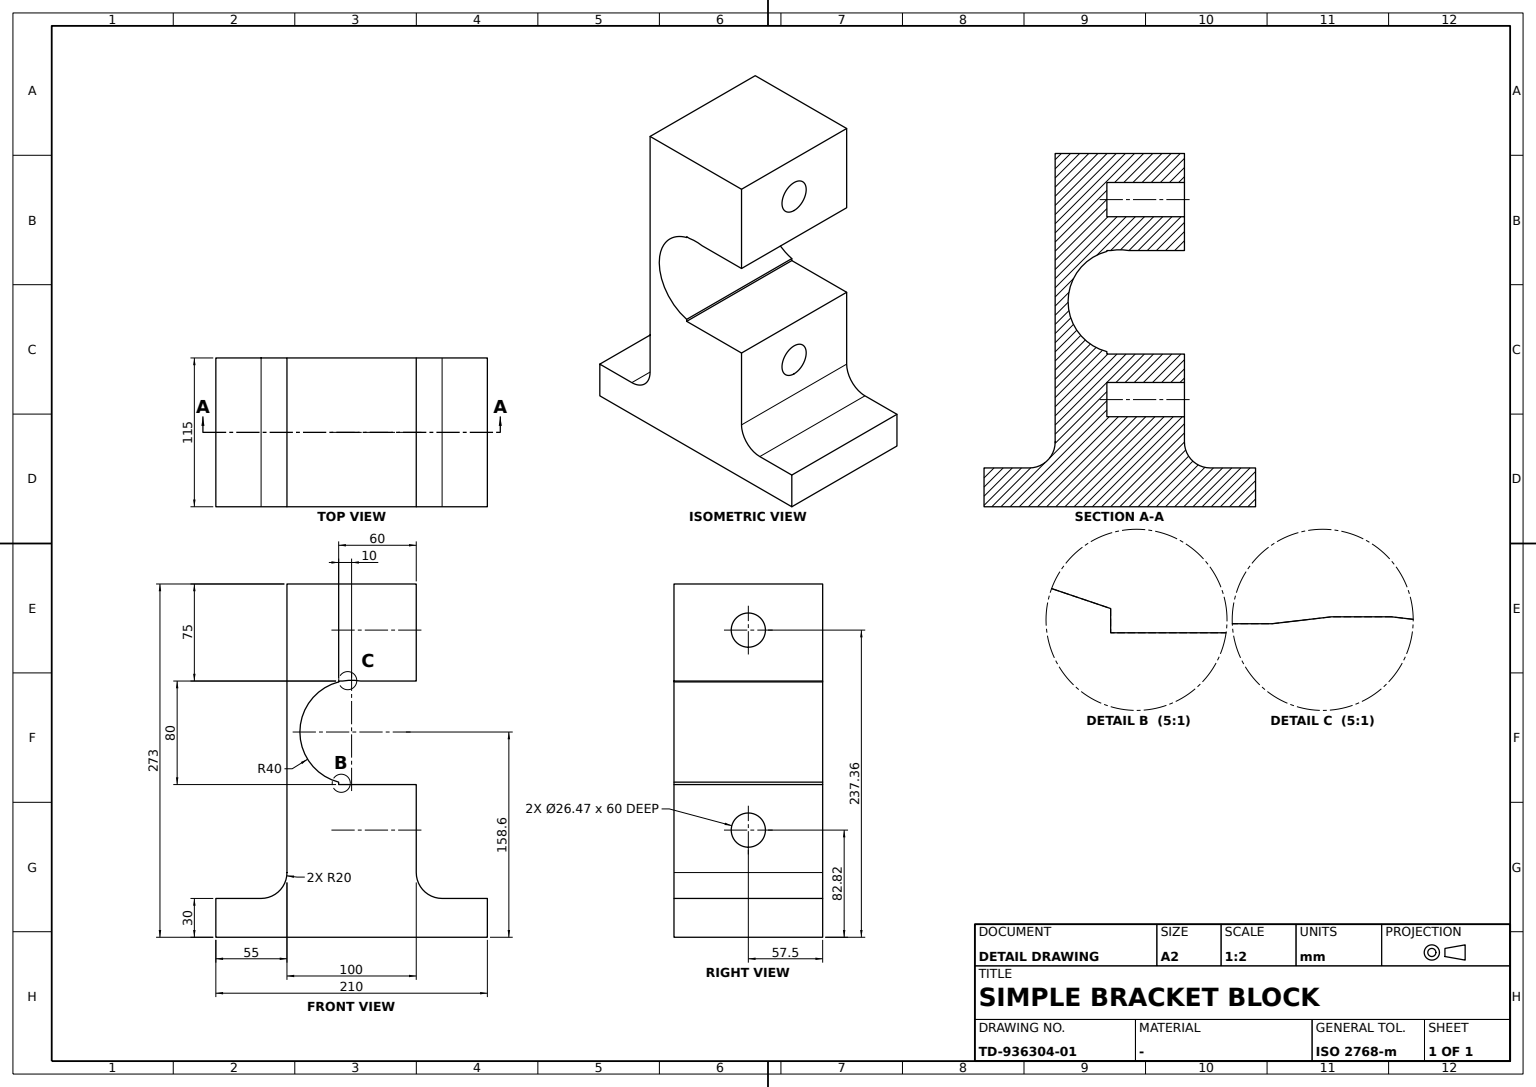
ISO-10303-21;
HEADER;
FILE_DESCRIPTION((''),'2;1');
FILE_NAME('','',(''),(''),'','','');
FILE_SCHEMA(('AUTOMOTIVE_DESIGN'));
ENDSEC;
DATA;
#1=APPLICATION_CONTEXT('');
#2=PRODUCT_CONTEXT('',#1,'mechanical');
#3=PRODUCT('','','',(#2));
#4=PRODUCT_DEFINITION_FORMATION('','',#3);
#5=PRODUCT_DEFINITION_CONTEXT('',#1,'design');
#6=PRODUCT_DEFINITION('','',#4,#5);
#7=PRODUCT_DEFINITION_SHAPE('','',#6);
#8=(LENGTH_UNIT()NAMED_UNIT(*)SI_UNIT(.MILLI.,.METRE.));
#9=(NAMED_UNIT(*)PLANE_ANGLE_UNIT()SI_UNIT($,.RADIAN.));
#10=(NAMED_UNIT(*)SI_UNIT($,.STERADIAN.)SOLID_ANGLE_UNIT());
#11=UNCERTAINTY_MEASURE_WITH_UNIT(LENGTH_MEASURE(0.005),#8,'distance_accuracy_value','');
#12=(GEOMETRIC_REPRESENTATION_CONTEXT(3)GLOBAL_UNCERTAINTY_ASSIGNED_CONTEXT((#11))GLOBAL_UNIT_ASSIGNED_CONTEXT((#8,#9,#10))REPRESENTATION_CONTEXT('',''));
#13=CARTESIAN_POINT('',(50.,57.5,118.));
#14=VERTEX_POINT('',#13);
#15=CARTESIAN_POINT('',(-10.,57.5,118.));
#16=VERTEX_POINT('',#15);
#17=DIRECTION('',(-1.,0.,0.));
#18=VECTOR('',#17,1000.);
#19=LINE('',#13,#18);
#20=EDGE_CURVE('',#14,#16,#19,.T.);
#21=ORIENTED_EDGE('',*,*,#20,.T.);
#22=CARTESIAN_POINT('',(-10.,-57.5,118.));
#23=VERTEX_POINT('',#22);
#24=DIRECTION('',(0.,-1.,0.));
#25=VECTOR('',#24,1000.);
#26=LINE('',#15,#25);
#27=EDGE_CURVE('',#16,#23,#26,.T.);
#28=ORIENTED_EDGE('',*,*,#27,.T.);
#29=CARTESIAN_POINT('',(50.,-57.5,118.));
#30=VERTEX_POINT('',#29);
#31=CARTESIAN_POINT('',(105.,-57.5,118.));
#32=LINE('',#31,#18);
#33=EDGE_CURVE('',#30,#23,#32,.T.);
#34=ORIENTED_EDGE('',*,*,#33,.F.);
#35=LINE('',#13,#25);
#36=EDGE_CURVE('',#14,#30,#35,.T.);
#37=ORIENTED_EDGE('',*,*,#36,.F.);
#38=EDGE_LOOP('',(#21,#28,#34,#37));
#39=FACE_BOUND('',#38,.T.);
#40=DIRECTION('',(0.,0.,-1.));
#41=AXIS2_PLACEMENT_3D('',#13,#40,#24);
#42=PLANE('',#41);
#43=ADVANCED_FACE('',(#39),#42,.F.);
#44=CARTESIAN_POINT('',(-105.,-57.5,0.));
#45=VERTEX_POINT('',#44);
#46=CARTESIAN_POINT('',(-105.,57.5,0.));
#47=VERTEX_POINT('',#46);
#48=CARTESIAN_POINT('',(-105.,0.,0.));
#49=DIRECTION('',(0.,1.,0.));
#50=VECTOR('',#49,1000.);
#51=LINE('',#48,#50);
#52=EDGE_CURVE('',#45,#47,#51,.T.);
#53=ORIENTED_EDGE('',*,*,#52,.F.);
#54=CARTESIAN_POINT('',(-105.,-57.5,30.));
#55=VERTEX_POINT('',#54);
#56=DIRECTION('',(0.,0.,1.));
#57=VECTOR('',#56,1000.);
#58=LINE('',#44,#57);
#59=EDGE_CURVE('',#45,#55,#58,.T.);
#60=ORIENTED_EDGE('',*,*,#59,.T.);
#61=CARTESIAN_POINT('',(-105.,57.5,30.));
#62=VERTEX_POINT('',#61);
#63=CARTESIAN_POINT('',(-105.,0.,30.));
#64=LINE('',#63,#50);
#65=EDGE_CURVE('',#55,#62,#64,.T.);
#66=ORIENTED_EDGE('',*,*,#65,.T.);
#67=LINE('',#46,#57);
#68=EDGE_CURVE('',#47,#62,#67,.T.);
#69=ORIENTED_EDGE('',*,*,#68,.F.);
#70=EDGE_LOOP('',(#53,#60,#66,#69));
#71=FACE_BOUND('',#70,.T.);
#72=DIRECTION('',(1.,0.,0.));
#73=AXIS2_PLACEMENT_3D('',#44,#72,#49);
#74=PLANE('',#73);
#75=ADVANCED_FACE('',(#71),#74,.F.);
#76=CARTESIAN_POINT('',(-50.,-57.5,50.));
#77=VERTEX_POINT('',#76);
#78=CARTESIAN_POINT('',(-50.,57.5,50.));
#79=VERTEX_POINT('',#78);
#80=CARTESIAN_POINT('',(-50.,0.,50.));
#81=LINE('',#80,#50);
#82=EDGE_CURVE('',#77,#79,#81,.T.);
#83=ORIENTED_EDGE('',*,*,#82,.F.);
#84=CARTESIAN_POINT('',(-50.,-57.5,273.));
#85=VERTEX_POINT('',#84);
#86=CARTESIAN_POINT('',(-50.,-57.5,30.));
#87=LINE('',#86,#57);
#88=EDGE_CURVE('',#77,#85,#87,.T.);
#89=ORIENTED_EDGE('',*,*,#88,.T.);
#90=CARTESIAN_POINT('',(-50.,57.5,273.));
#91=VERTEX_POINT('',#90);
#92=CARTESIAN_POINT('',(-50.,0.,273.));
#93=LINE('',#92,#50);
#94=EDGE_CURVE('',#85,#91,#93,.T.);
#95=ORIENTED_EDGE('',*,*,#94,.T.);
#96=CARTESIAN_POINT('',(-50.,57.5,0.));
#97=LINE('',#96,#57);
#98=EDGE_CURVE('',#79,#91,#97,.T.);
#99=ORIENTED_EDGE('',*,*,#98,.F.);
#100=EDGE_LOOP('',(#83,#89,#95,#99));
#101=FACE_BOUND('',#100,.T.);
#102=AXIS2_PLACEMENT_3D('',#86,#72,#49);
#103=PLANE('',#102);
#104=ADVANCED_FACE('',(#101),#103,.F.);
#105=CARTESIAN_POINT('',(50.,57.5,50.));
#106=VERTEX_POINT('',#105);
#107=CARTESIAN_POINT('',(70.,57.5,30.));
#108=VERTEX_POINT('',#107);
#109=CARTESIAN_POINT('',(70.,57.5,50.));
#110=AXIS2_PLACEMENT_3D('',#109,#24,#40);
#111=CIRCLE('',#110,20.);
#112=EDGE_CURVE('',#106,#108,#111,.T.);
#113=ORIENTED_EDGE('',*,*,#112,.F.);
#114=CARTESIAN_POINT('',(50.,-57.5,50.));
#115=VERTEX_POINT('',#114);
#116=CARTESIAN_POINT('',(50.,0.,50.));
#117=LINE('',#116,#25);
#118=EDGE_CURVE('',#106,#115,#117,.T.);
#119=ORIENTED_EDGE('',*,*,#118,.T.);
#120=CARTESIAN_POINT('',(70.,-57.5,30.));
#121=VERTEX_POINT('',#120);
#122=CARTESIAN_POINT('',(70.,-57.5,50.));
#123=AXIS2_PLACEMENT_3D('',#122,#49,#56);
#124=CIRCLE('',#123,20.);
#125=EDGE_CURVE('',#121,#115,#124,.T.);
#126=ORIENTED_EDGE('',*,*,#125,.F.);
#127=CARTESIAN_POINT('',(70.,0.,30.));
#128=LINE('',#127,#25);
#129=EDGE_CURVE('',#108,#121,#128,.T.);
#130=ORIENTED_EDGE('',*,*,#129,.F.);
#131=EDGE_LOOP('',(#113,#119,#126,#130));
#132=FACE_BOUND('',#131,.T.);
#133=CARTESIAN_POINT('',(70.,0.,50.));
#134=AXIS2_PLACEMENT_3D('',#133,#24,#40);
#135=CYLINDRICAL_SURFACE('',#134,20.);
#136=ADVANCED_FACE('',(#132),#135,.F.);
#137=CARTESIAN_POINT('',(6.915696,-57.5,198.));
#138=VERTEX_POINT('',#137);
#139=CARTESIAN_POINT('',(6.915696,57.5,198.));
#140=VERTEX_POINT('',#139);
#141=LINE('',#139,#50);
#142=EDGE_CURVE('',#138,#140,#141,.T.);
#143=ORIENTED_EDGE('',*,*,#142,.F.);
#144=CARTESIAN_POINT('',(-6.915696,-57.5,198.));
#145=VERTEX_POINT('',#144);
#146=CARTESIAN_POINT('',(0.,-57.5,158.602371));
#147=AXIS2_PLACEMENT_3D('',#146,#49,#56);
#148=CIRCLE('',#147,40.);
#149=EDGE_CURVE('',#145,#138,#148,.T.);
#150=ORIENTED_EDGE('',*,*,#149,.F.);
#151=CARTESIAN_POINT('',(-6.915696,57.5,198.));
#152=VERTEX_POINT('',#151);
#153=LINE('',#151,#50);
#154=EDGE_CURVE('',#152,#145,#153,.F.);
#155=ORIENTED_EDGE('',*,*,#154,.F.);
#156=CARTESIAN_POINT('',(0.,57.5,158.602371));
#157=AXIS2_PLACEMENT_3D('',#156,#24,#40);
#158=CIRCLE('',#157,40.);
#159=EDGE_CURVE('',#152,#140,#158,.F.);
#160=ORIENTED_EDGE('',*,*,#159,.T.);
#161=EDGE_LOOP('',(#143,#150,#155,#160));
#162=FACE_BOUND('',#161,.T.);
#163=CARTESIAN_POINT('',(0.,-0.66,158.602371));
#164=AXIS2_PLACEMENT_3D('',#163,#49,#17);
#165=CYLINDRICAL_SURFACE('',#164,40.);
#166=ADVANCED_FACE('',(#162),#165,.F.);
#167=ORIENTED_EDGE('',*,*,#129,.T.);
#168=CARTESIAN_POINT('',(105.,-57.5,30.));
#169=VERTEX_POINT('',#168);
#170=CARTESIAN_POINT('',(0.,-57.5,30.));
#171=LINE('',#170,#18);
#172=EDGE_CURVE('',#169,#121,#171,.T.);
#173=ORIENTED_EDGE('',*,*,#172,.F.);
#174=CARTESIAN_POINT('',(105.,57.5,30.));
#175=VERTEX_POINT('',#174);
#176=CARTESIAN_POINT('',(105.,0.,30.));
#177=LINE('',#176,#25);
#178=EDGE_CURVE('',#175,#169,#177,.T.);
#179=ORIENTED_EDGE('',*,*,#178,.F.);
#180=CARTESIAN_POINT('',(0.,57.5,30.));
#181=VECTOR('',#72,1000.);
#182=LINE('',#180,#181);
#183=EDGE_CURVE('',#108,#175,#182,.T.);
#184=ORIENTED_EDGE('',*,*,#183,.F.);
#185=EDGE_LOOP('',(#167,#173,#179,#184));
#186=FACE_BOUND('',#185,.T.);
#187=CARTESIAN_POINT('',(0.,0.,30.));
#188=AXIS2_PLACEMENT_3D('',#187,#56,#72);
#189=PLANE('',#188);
#190=ADVANCED_FACE('',(#186),#189,.T.);
#191=CARTESIAN_POINT('',(-10.,0.,224.12904));
#192=VERTEX_POINT('',#191);
#193=CARTESIAN_POINT('',(-10.,0.,237.361694));
#194=AXIS2_PLACEMENT_3D('',#193,#72,#40);
#195=CIRCLE('',#194,13.232654);
#196=EDGE_CURVE('',#192,#192,#195,.T.);
#197=ORIENTED_EDGE('',*,*,#196,.T.);
#198=EDGE_LOOP('',(#197));
#199=FACE_BOUND('',#198,.T.);
#200=CARTESIAN_POINT('',(-10.,0.,0.));
#201=AXIS2_PLACEMENT_3D('',#200,#72,#49);
#202=PLANE('',#201);
#203=ADVANCED_FACE('',(#199),#202,.T.);
#204=CARTESIAN_POINT('',(-70.,-57.5,30.));
#205=VERTEX_POINT('',#204);
#206=CARTESIAN_POINT('',(-70.,57.5,30.));
#207=VERTEX_POINT('',#206);
#208=CARTESIAN_POINT('',(-70.,0.,30.));
#209=LINE('',#208,#50);
#210=EDGE_CURVE('',#205,#207,#209,.T.);
#211=ORIENTED_EDGE('',*,*,#210,.T.);
#212=EDGE_CURVE('',#62,#207,#182,.T.);
#213=ORIENTED_EDGE('',*,*,#212,.F.);
#214=ORIENTED_EDGE('',*,*,#65,.F.);
#215=EDGE_CURVE('',#205,#55,#171,.T.);
#216=ORIENTED_EDGE('',*,*,#215,.F.);
#217=EDGE_LOOP('',(#211,#213,#214,#216));
#218=FACE_BOUND('',#217,.T.);
#219=ADVANCED_FACE('',(#218),#189,.T.);
#220=CARTESIAN_POINT('',(50.,0.,250.594349));
#221=VERTEX_POINT('',#220);
#222=CARTESIAN_POINT('',(50.,0.,237.361694));
#223=AXIS2_PLACEMENT_3D('',#222,#17,#56);
#224=CIRCLE('',#223,13.232654);
#225=EDGE_CURVE('',#221,#221,#224,.F.);
#226=ORIENTED_EDGE('',*,*,#225,.T.);
#227=EDGE_LOOP('',(#226));
#228=FACE_BOUND('',#227,.T.);
#229=ORIENTED_EDGE('',*,*,#196,.F.);
#230=EDGE_LOOP('',(#229));
#231=FACE_BOUND('',#230,.T.);
#232=CARTESIAN_POINT('',(20.,0.,237.361694));
#233=AXIS2_PLACEMENT_3D('',#232,#72,#49);
#234=CYLINDRICAL_SURFACE('',#233,13.232654);
#235=ADVANCED_FACE('',(#228,#231),#234,.F.);
#236=ORIENTED_EDGE('',*,*,#178,.T.);
#237=CARTESIAN_POINT('',(105.,-57.5,0.));
#238=VERTEX_POINT('',#237);
#239=LINE('',#237,#57);
#240=EDGE_CURVE('',#238,#169,#239,.T.);
#241=ORIENTED_EDGE('',*,*,#240,.F.);
#242=CARTESIAN_POINT('',(105.,57.5,0.));
#243=VERTEX_POINT('',#242);
#244=CARTESIAN_POINT('',(105.,0.,0.));
#245=LINE('',#244,#25);
#246=EDGE_CURVE('',#243,#238,#245,.T.);
#247=ORIENTED_EDGE('',*,*,#246,.F.);
#248=LINE('',#242,#57);
#249=EDGE_CURVE('',#243,#175,#248,.T.);
#250=ORIENTED_EDGE('',*,*,#249,.T.);
#251=EDGE_LOOP('',(#236,#241,#247,#250));
#252=FACE_BOUND('',#251,.T.);
#253=AXIS2_PLACEMENT_3D('',#242,#17,#24);
#254=PLANE('',#253);
#255=ADVANCED_FACE('',(#252),#254,.F.);
#256=CARTESIAN_POINT('',(-70.,57.5,50.));
#257=AXIS2_PLACEMENT_3D('',#256,#24,#40);
#258=CIRCLE('',#257,20.);
#259=EDGE_CURVE('',#207,#79,#258,.T.);
#260=ORIENTED_EDGE('',*,*,#259,.F.);
#261=ORIENTED_EDGE('',*,*,#210,.F.);
#262=CARTESIAN_POINT('',(-70.,-57.5,50.));
#263=AXIS2_PLACEMENT_3D('',#262,#49,#56);
#264=CIRCLE('',#263,20.);
#265=EDGE_CURVE('',#77,#205,#264,.T.);
#266=ORIENTED_EDGE('',*,*,#265,.F.);
#267=ORIENTED_EDGE('',*,*,#82,.T.);
#268=EDGE_LOOP('',(#260,#261,#266,#267));
#269=FACE_BOUND('',#268,.T.);
#270=CARTESIAN_POINT('',(-70.,0.,50.));
#271=AXIS2_PLACEMENT_3D('',#270,#49,#40);
#272=CYLINDRICAL_SURFACE('',#271,20.);
#273=ADVANCED_FACE('',(#269),#272,.F.);
#274=CARTESIAN_POINT('',(-10.,0.000177,69.582562));
#275=VERTEX_POINT('',#274);
#276=CARTESIAN_POINT('',(-10.,0.000177,82.815216));
#277=AXIS2_PLACEMENT_3D('',#276,#72,#40);
#278=CIRCLE('',#277,13.232654);
#279=EDGE_CURVE('',#275,#275,#278,.T.);
#280=ORIENTED_EDGE('',*,*,#279,.F.);
#281=EDGE_LOOP('',(#280));
#282=FACE_BOUND('',#281,.T.);
#283=CARTESIAN_POINT('',(50.,0.000177,96.04787));
#284=VERTEX_POINT('',#283);
#285=CARTESIAN_POINT('',(50.,0.000177,82.815216));
#286=AXIS2_PLACEMENT_3D('',#285,#17,#56);
#287=CIRCLE('',#286,13.232654);
#288=EDGE_CURVE('',#284,#284,#287,.F.);
#289=ORIENTED_EDGE('',*,*,#288,.T.);
#290=EDGE_LOOP('',(#289));
#291=FACE_BOUND('',#290,.T.);
#292=CARTESIAN_POINT('',(20.,0.000177,82.815216));
#293=AXIS2_PLACEMENT_3D('',#292,#72,#49);
#294=CYLINDRICAL_SURFACE('',#293,13.232654);
#295=ADVANCED_FACE('',(#282,#291),#294,.F.);
#296=ORIENTED_EDGE('',*,*,#94,.F.);
#297=CARTESIAN_POINT('',(50.,-57.5,273.));
#298=VERTEX_POINT('',#297);
#299=CARTESIAN_POINT('',(0.,-57.5,273.));
#300=LINE('',#299,#18);
#301=EDGE_CURVE('',#298,#85,#300,.T.);
#302=ORIENTED_EDGE('',*,*,#301,.F.);
#303=CARTESIAN_POINT('',(50.,57.5,273.));
#304=VERTEX_POINT('',#303);
#305=CARTESIAN_POINT('',(50.,0.,273.));
#306=LINE('',#305,#25);
#307=EDGE_CURVE('',#304,#298,#306,.T.);
#308=ORIENTED_EDGE('',*,*,#307,.F.);
#309=CARTESIAN_POINT('',(0.,57.5,273.));
#310=LINE('',#309,#181);
#311=EDGE_CURVE('',#91,#304,#310,.T.);
#312=ORIENTED_EDGE('',*,*,#311,.F.);
#313=EDGE_LOOP('',(#296,#302,#308,#312));
#314=FACE_BOUND('',#313,.T.);
#315=CARTESIAN_POINT('',(0.,0.,273.));
#316=AXIS2_PLACEMENT_3D('',#315,#56,#72);
#317=PLANE('',#316);
#318=ADVANCED_FACE('',(#314),#317,.T.);
#319=CARTESIAN_POINT('',(50.,57.5,198.));
#320=VERTEX_POINT('',#319);
#321=CARTESIAN_POINT('',(-105.,57.5,198.));
#322=LINE('',#321,#18);
#323=EDGE_CURVE('',#320,#140,#322,.T.);
#324=ORIENTED_EDGE('',*,*,#323,.F.);
#325=CARTESIAN_POINT('',(50.,-57.5,198.));
#326=VERTEX_POINT('',#325);
#327=LINE('',#319,#50);
#328=EDGE_CURVE('',#326,#320,#327,.T.);
#329=ORIENTED_EDGE('',*,*,#328,.F.);
#330=LINE('',#325,#18);
#331=EDGE_CURVE('',#326,#138,#330,.T.);
#332=ORIENTED_EDGE('',*,*,#331,.T.);
#333=ORIENTED_EDGE('',*,*,#142,.T.);
#334=EDGE_LOOP('',(#324,#329,#332,#333));
#335=FACE_BOUND('',#334,.T.);
#336=AXIS2_PLACEMENT_3D('',#325,#56,#49);
#337=PLANE('',#336);
#338=ADVANCED_FACE('',(#335),#337,.F.);
#339=ORIENTED_EDGE('',*,*,#112,.T.);
#340=ORIENTED_EDGE('',*,*,#183,.T.);
#341=ORIENTED_EDGE('',*,*,#249,.F.);
#342=CARTESIAN_POINT('',(0.,57.5,0.));
#343=LINE('',#342,#181);
#344=EDGE_CURVE('',#47,#243,#343,.T.);
#345=ORIENTED_EDGE('',*,*,#344,.F.);
#346=ORIENTED_EDGE('',*,*,#68,.T.);
#347=ORIENTED_EDGE('',*,*,#212,.T.);
#348=ORIENTED_EDGE('',*,*,#259,.T.);
#349=ORIENTED_EDGE('',*,*,#98,.T.);
#350=ORIENTED_EDGE('',*,*,#311,.T.);
#351=CARTESIAN_POINT('',(50.,57.5,30.));
#352=LINE('',#351,#57);
#353=EDGE_CURVE('',#320,#304,#352,.T.);
#354=ORIENTED_EDGE('',*,*,#353,.F.);
#355=ORIENTED_EDGE('',*,*,#323,.T.);
#356=ORIENTED_EDGE('',*,*,#159,.F.);
#357=CARTESIAN_POINT('',(-10.,57.5,198.));
#358=VERTEX_POINT('',#357);
#359=EDGE_CURVE('',#152,#358,#322,.T.);
#360=ORIENTED_EDGE('',*,*,#359,.T.);
#361=CARTESIAN_POINT('',(-10.,57.5,197.332205));
#362=VERTEX_POINT('',#361);
#363=CARTESIAN_POINT('',(-10.,57.5,0.));
#364=VECTOR('',#40,1000.);
#365=LINE('',#363,#364);
#366=EDGE_CURVE('',#358,#362,#365,.T.);
#367=ORIENTED_EDGE('',*,*,#366,.T.);
#368=CARTESIAN_POINT('',(-10.,57.5,119.872538));
#369=VERTEX_POINT('',#368);
#370=EDGE_CURVE('',#369,#362,#158,.F.);
#371=ORIENTED_EDGE('',*,*,#370,.F.);
#372=EDGE_CURVE('',#369,#16,#365,.T.);
#373=ORIENTED_EDGE('',*,*,#372,.T.);
#374=ORIENTED_EDGE('',*,*,#20,.F.);
#375=EDGE_CURVE('',#106,#14,#352,.T.);
#376=ORIENTED_EDGE('',*,*,#375,.F.);
#377=EDGE_LOOP('',(#339,#340,#341,#345,#346,#347,#348,#349,#350,#354,#355,#356,#360,#367,#371,#373,#374,#376));
#378=FACE_BOUND('',#377,.T.);
#379=AXIS2_PLACEMENT_3D('',#46,#24,#72);
#380=PLANE('',#379);
#381=ADVANCED_FACE('',(#378),#380,.F.);
#382=ORIENTED_EDGE('',*,*,#279,.T.);
#383=EDGE_LOOP('',(#382));
#384=FACE_BOUND('',#383,.T.);
#385=ADVANCED_FACE('',(#384),#202,.T.);
#386=ORIENTED_EDGE('',*,*,#225,.F.);
#387=EDGE_LOOP('',(#386));
#388=FACE_BOUND('',#387,.T.);
#389=ORIENTED_EDGE('',*,*,#307,.T.);
#390=CARTESIAN_POINT('',(50.,-57.5,0.));
#391=LINE('',#390,#57);
#392=EDGE_CURVE('',#326,#298,#391,.T.);
#393=ORIENTED_EDGE('',*,*,#392,.F.);
#394=ORIENTED_EDGE('',*,*,#328,.T.);
#395=ORIENTED_EDGE('',*,*,#353,.T.);
#396=EDGE_LOOP('',(#389,#393,#394,#395));
#397=FACE_BOUND('',#396,.T.);
#398=AXIS2_PLACEMENT_3D('',#351,#17,#24);
#399=PLANE('',#398);
#400=ADVANCED_FACE('',(#388,#397),#399,.F.);
#401=CARTESIAN_POINT('',(-10.,-57.5,197.332205));
#402=VERTEX_POINT('',#401);
#403=CARTESIAN_POINT('',(-10.,-57.5,198.));
#404=VERTEX_POINT('',#403);
#405=CARTESIAN_POINT('',(-10.,-57.5,0.));
#406=LINE('',#405,#57);
#407=EDGE_CURVE('',#402,#404,#406,.T.);
#408=ORIENTED_EDGE('',*,*,#407,.F.);
#409=LINE('',#361,#50);
#410=EDGE_CURVE('',#402,#362,#409,.T.);
#411=ORIENTED_EDGE('',*,*,#410,.T.);
#412=ORIENTED_EDGE('',*,*,#366,.F.);
#413=LINE('',#403,#50);
#414=EDGE_CURVE('',#404,#358,#413,.T.);
#415=ORIENTED_EDGE('',*,*,#414,.F.);
#416=EDGE_LOOP('',(#408,#411,#412,#415));
#417=FACE_BOUND('',#416,.T.);
#418=ADVANCED_FACE('',(#417),#202,.T.);
#419=CARTESIAN_POINT('',(0.,-57.5,0.));
#420=LINE('',#419,#18);
#421=EDGE_CURVE('',#238,#45,#420,.T.);
#422=ORIENTED_EDGE('',*,*,#421,.T.);
#423=ORIENTED_EDGE('',*,*,#52,.T.);
#424=ORIENTED_EDGE('',*,*,#344,.T.);
#425=ORIENTED_EDGE('',*,*,#246,.T.);
#426=EDGE_LOOP('',(#422,#423,#424,#425));
#427=FACE_BOUND('',#426,.T.);
#428=CARTESIAN_POINT('',(0.,0.,0.));
#429=AXIS2_PLACEMENT_3D('',#428,#56,#72);
#430=PLANE('',#429);
#431=ADVANCED_FACE('',(#427),#430,.F.);
#432=ORIENTED_EDGE('',*,*,#88,.F.);
#433=ORIENTED_EDGE('',*,*,#265,.T.);
#434=ORIENTED_EDGE('',*,*,#215,.T.);
#435=ORIENTED_EDGE('',*,*,#59,.F.);
#436=ORIENTED_EDGE('',*,*,#421,.F.);
#437=ORIENTED_EDGE('',*,*,#240,.T.);
#438=ORIENTED_EDGE('',*,*,#172,.T.);
#439=ORIENTED_EDGE('',*,*,#125,.T.);
#440=EDGE_CURVE('',#115,#30,#391,.T.);
#441=ORIENTED_EDGE('',*,*,#440,.T.);
#442=ORIENTED_EDGE('',*,*,#33,.T.);
#443=CARTESIAN_POINT('',(-10.,-57.5,119.872538));
#444=VERTEX_POINT('',#443);
#445=EDGE_CURVE('',#23,#444,#406,.T.);
#446=ORIENTED_EDGE('',*,*,#445,.T.);
#447=EDGE_CURVE('',#444,#402,#148,.T.);
#448=ORIENTED_EDGE('',*,*,#447,.T.);
#449=ORIENTED_EDGE('',*,*,#407,.T.);
#450=EDGE_CURVE('',#145,#404,#330,.T.);
#451=ORIENTED_EDGE('',*,*,#450,.F.);
#452=ORIENTED_EDGE('',*,*,#149,.T.);
#453=ORIENTED_EDGE('',*,*,#331,.F.);
#454=ORIENTED_EDGE('',*,*,#392,.T.);
#455=ORIENTED_EDGE('',*,*,#301,.T.);
#456=EDGE_LOOP('',(#432,#433,#434,#435,#436,#437,#438,#439,#441,#442,#446,#448,#449,#451,#452,#453,#454,#455));
#457=FACE_BOUND('',#456,.T.);
#458=AXIS2_PLACEMENT_3D('',#237,#49,#17);
#459=PLANE('',#458);
#460=ADVANCED_FACE('',(#457),#459,.F.);
#461=ORIENTED_EDGE('',*,*,#410,.F.);
#462=ORIENTED_EDGE('',*,*,#447,.F.);
#463=LINE('',#368,#50);
#464=EDGE_CURVE('',#369,#444,#463,.F.);
#465=ORIENTED_EDGE('',*,*,#464,.F.);
#466=ORIENTED_EDGE('',*,*,#370,.T.);
#467=EDGE_LOOP('',(#461,#462,#465,#466));
#468=FACE_BOUND('',#467,.T.);
#469=ADVANCED_FACE('',(#468),#165,.F.);
#470=ORIENTED_EDGE('',*,*,#36,.T.);
#471=ORIENTED_EDGE('',*,*,#440,.F.);
#472=ORIENTED_EDGE('',*,*,#118,.F.);
#473=ORIENTED_EDGE('',*,*,#375,.T.);
#474=EDGE_LOOP('',(#470,#471,#472,#473));
#475=FACE_BOUND('',#474,.T.);
#476=ORIENTED_EDGE('',*,*,#288,.F.);
#477=EDGE_LOOP('',(#476));
#478=FACE_BOUND('',#477,.T.);
#479=ADVANCED_FACE('',(#475,#478),#399,.F.);
#480=ORIENTED_EDGE('',*,*,#414,.T.);
#481=ORIENTED_EDGE('',*,*,#359,.F.);
#482=ORIENTED_EDGE('',*,*,#154,.T.);
#483=ORIENTED_EDGE('',*,*,#450,.T.);
#484=EDGE_LOOP('',(#480,#481,#482,#483));
#485=FACE_BOUND('',#484,.T.);
#486=ADVANCED_FACE('',(#485),#337,.F.);
#487=ORIENTED_EDGE('',*,*,#464,.T.);
#488=ORIENTED_EDGE('',*,*,#445,.F.);
#489=ORIENTED_EDGE('',*,*,#27,.F.);
#490=ORIENTED_EDGE('',*,*,#372,.F.);
#491=EDGE_LOOP('',(#487,#488,#489,#490));
#492=FACE_BOUND('',#491,.T.);
#493=ADVANCED_FACE('',(#492),#202,.T.);
#494=CLOSED_SHELL('',(#43,#75,#104,#136,#166,#190,#203,#219,#235,#255,#273,#295,#318,#338,#381,#385,#400,#418,#431,#460,#469,#479,#486,#493));
#495=MANIFOLD_SOLID_BREP('',#494);
#496=ADVANCED_BREP_SHAPE_REPRESENTATION('',(#495),#12);
#497=SHAPE_DEFINITION_REPRESENTATION(#7,#496);
ENDSEC;
END-ISO-10303-21;
